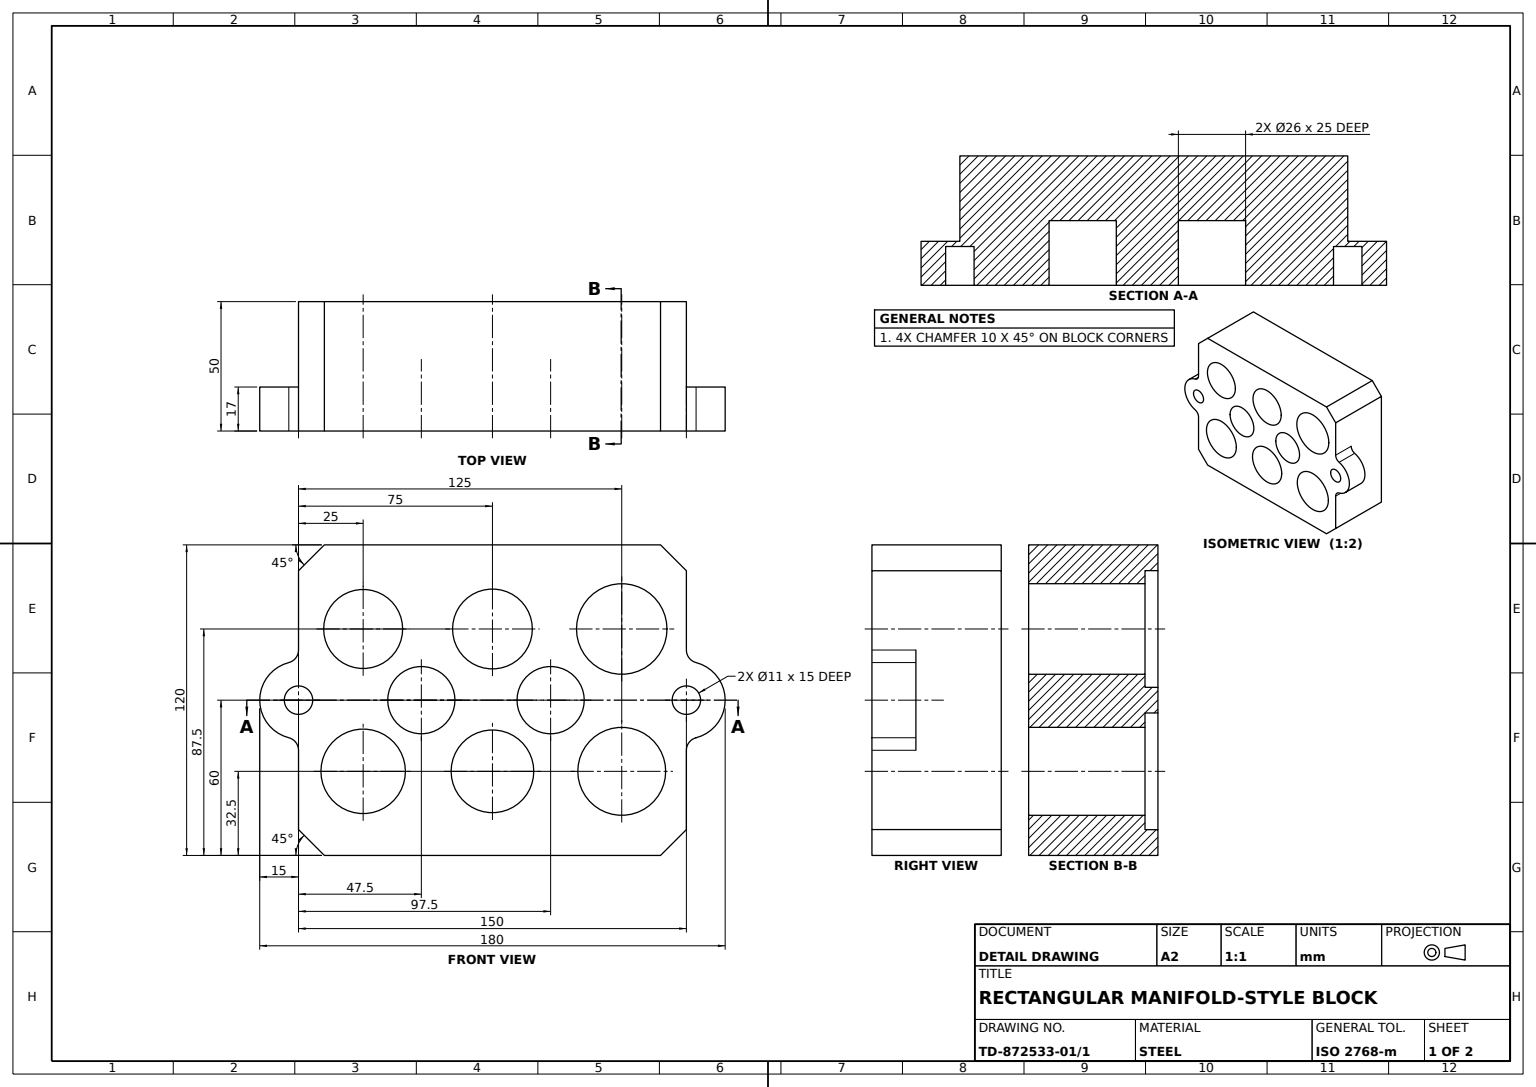
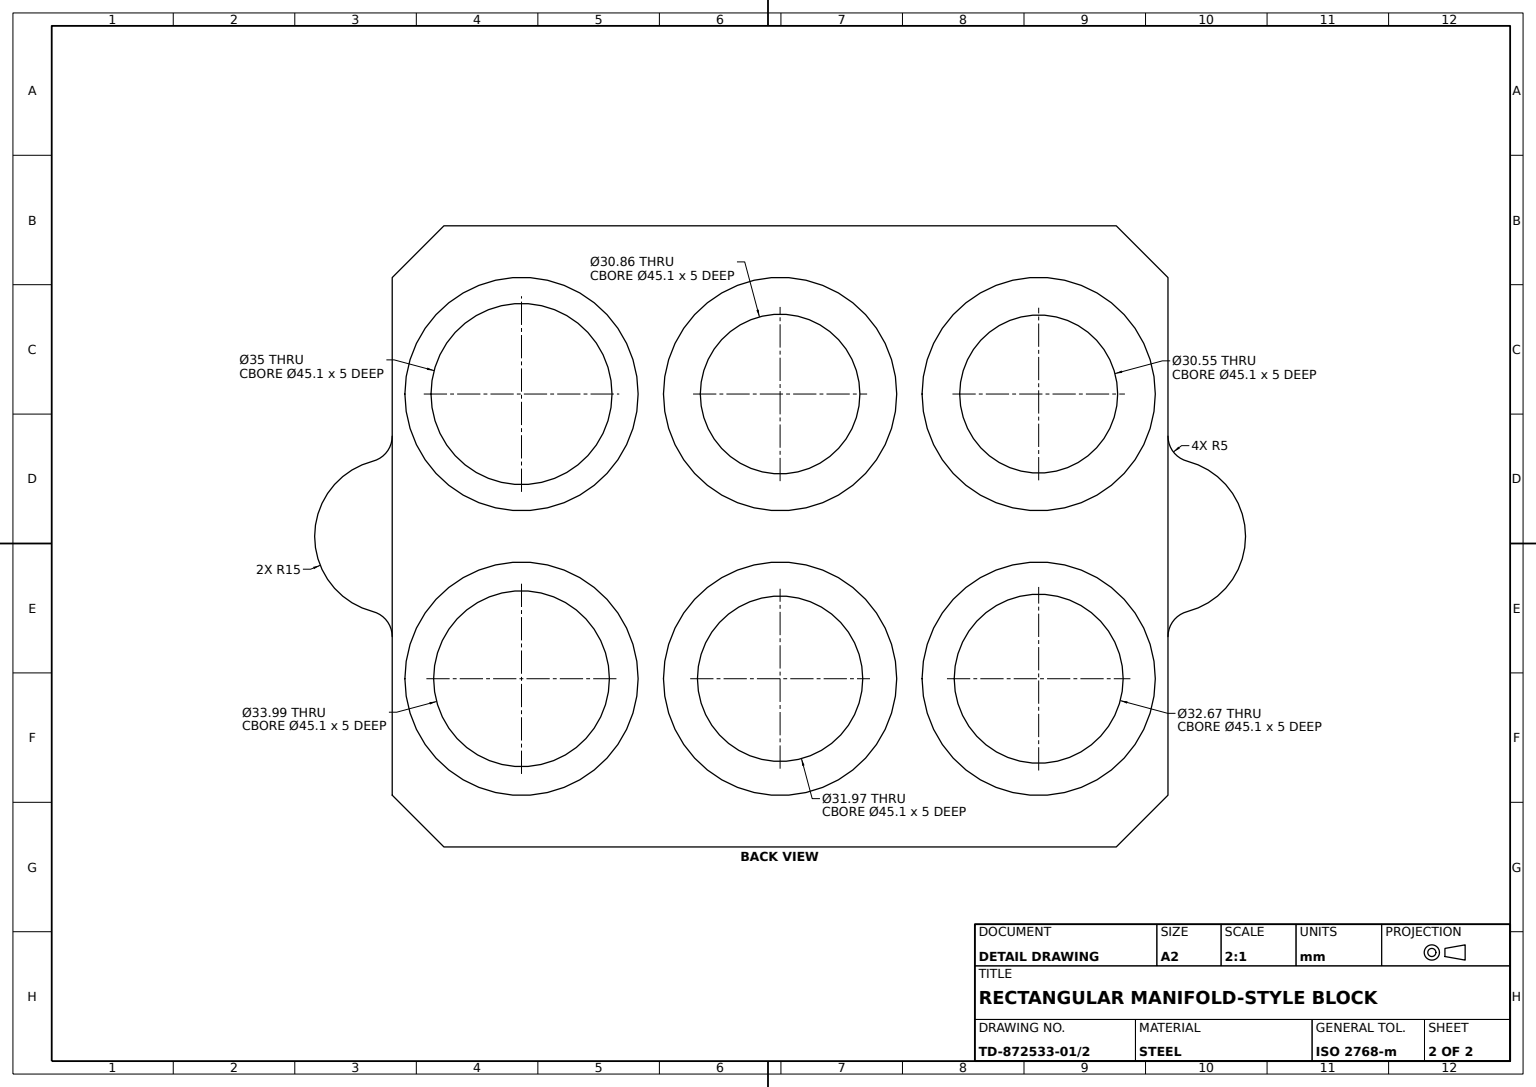
solid
v1 (153.75,74.523688,33)
v2 (150,79.364917,33)
e1 v1 v2 CIRCLE(AX(P(155,79.364917,33),D(0,0,-1),D(-1,0,0)),5)
v3 (165,60,33)
e2 v3 v1 CIRCLE(AX(P(150,60,33),D(0,0,1),D(-1,0,0)),15)
v4 (153.75,45.476312,33)
e3 v4 v3 CIRCLE(AX(P(150,60,33),D(0,0,1),D(-1,0,0)),15)
v5 (150,40.635083,33)
e4 v5 v4 CIRCLE(AX(P(155,40.635083,33),D(0,0,-1),D(1,0,0)),5)
e5 v2 v5 LINE
face PLANE(AX(P(150,60,33),D(0,0,-1),D(-1,0,0))) [-e1 -e2 -e3 -e4 -e5]
v6 (150,79.364917,50)
e6 v2 v6 LINE
v7 (150,40.635083,50)
e7 v5 v7 LINE
v8 (150,10,50)
e8 v8 v7 LINE
v9 (150,10,0)
e9 v8 v9 LINE
v10 (150,110,0)
e10 v9 v10 LINE
v11 (150,110,50)
e11 v10 v11 LINE
e12 v6 v11 LINE
face PLANE(AX(P(150,0,50),D(-1,0,0),D(0,0,1))) rev [-e6 e5 e7 -e8 e9 e10 e11 -e12]
v12 (142.5,87.5,50)
v13 (142.5,87.5,5)
e13 v12 v13 LINE
v14 (107.5,87.5,50)
e14 v14 v12 CIRCLE(AX(P(125,87.5,50),D(0,0,-1),D(-1,0,0)),17.5)
v15 (107.5,87.5,5)
e15 v14 v15 LINE
e16 v15 v13 CIRCLE(AX(P(125,87.5,5),D(0,0,-1),D(-1,0,0)),17.5)
face CYL(AX(P(125,87.5,50),D(0,0,-1),D(-1,0,0)),17.5) rev [-e13 -e14 e15 e16]
v16 (-5.5,60,35)
v17 (5.5,60,35)
e17 v16 v17 CIRCLE(AX(P(0,60,35),D(0,0,1),D(1,0,0)),5.5)
e18 v17 v16 CIRCLE(AX(P(0,60,35),D(0,0,1),D(1,0,0)),5.5)
face PLANE(AX(P(0,60,35),D(0,0,1),D(1,0,0))) [e17 e18]
v18 (2.45,87.5,5)
v19 (2.45,87.5,0)
e19 v18 v19 LINE
v20 (47.55,87.5,0)
e20 v19 v20 CIRCLE(AX(P(25,87.5,0),D(0,0,-1),D(-1,0,0)),22.55)
v21 (47.55,87.5,5)
e21 v21 v20 LINE
e22 v18 v21 CIRCLE(AX(P(25,87.5,5),D(0,0,-1),D(-1,0,0)),22.55)
face CYL(AX(P(25,87.5,5),D(0,0,-1),D(-1,0,0)),22.55) rev [e19 e20 -e21 -e22]
v22 (141.993107,32.5,50)
v23 (108.006893,32.5,50)
e23 v22 v23 CIRCLE(AX(P(125,32.5,50),D(0,0,-1),D(-1,0,0)),16.993107)
v24 (141.993107,32.5,5)
e24 v22 v24 LINE
v25 (108.006893,32.5,5)
e25 v24 v25 CIRCLE(AX(P(125,32.5,5),D(0,0,-1),D(-1,0,0)),16.993107)
e26 v23 v25 LINE
face CYL(AX(P(125,32.5,50),D(0,0,-1),D(-1,0,0)),16.993107) rev [-e23 e24 e25 -e26]
v26 (9.725741,87.5,50)
v27 (40.274259,87.5,50)
e27 v26 v27 CIRCLE(AX(P(25,87.5,50),D(0,0,-1),D(-1,0,0)),15.274259)
v28 (9.725741,87.5,5)
e28 v26 v28 LINE
v29 (40.274259,87.5,5)
e29 v28 v29 CIRCLE(AX(P(25,87.5,5),D(0,0,-1),D(-1,0,0)),15.274259)
e30 v27 v29 LINE
face CYL(AX(P(25,87.5,50),D(0,0,-1),D(-1,0,0)),15.274259) rev [-e27 e28 e29 -e30]
v30 (2.45,32.5,0)
v31 (47.55,32.5,0)
e31 v30 v31 CIRCLE(AX(P(25,32.5,0),D(0,0,-1),D(-1,0,0)),22.55)
v32 (47.55,32.5,5)
e32 v32 v31 LINE
v33 (2.45,32.5,5)
e33 v33 v32 CIRCLE(AX(P(25,32.5,5),D(0,0,-1),D(-1,0,0)),22.55)
e34 v33 v30 LINE
face CYL(AX(P(25,32.5,5),D(0,0,-1),D(-1,0,0)),22.55) rev [e31 -e32 -e33 e34]
v34 (110.5,60,25)
v35 (110.5,60,50)
e35 v34 v35 LINE
v36 (84.5,60,25)
e36 v36 v34 CIRCLE(AX(P(97.5,60,25),D(0,0,1),D(1,0,0)),13)
v37 (84.5,60,50)
e37 v36 v37 LINE
e38 v37 v35 CIRCLE(AX(P(97.5,60,50),D(0,0,1),D(1,0,0)),13)
face CYL(AX(P(97.5,60,25),D(0,0,1),D(1,0,0)),13) rev [-e35 -e36 e37 e38]
v38 (5.5,60,50)
e39 v17 v38 LINE
v39 (-5.5,60,50)
e40 v38 v39 CIRCLE(AX(P(0,60,50),D(0,0,1),D(1,0,0)),5.5)
e41 v16 v39 LINE
face CYL(AX(P(0,60,35),D(0,0,1),D(1,0,0)),5.5) rev [-e18 e39 e40 -e41]
v40 (102.45,87.5,5)
v41 (147.55,87.5,5)
e42 v40 v41 CIRCLE(AX(P(125,87.5,5),D(0,0,-1),D(-1,0,0)),22.55)
v42 (102.45,87.5,0)
e43 v40 v42 LINE
v43 (147.55,87.5,0)
e44 v42 v43 CIRCLE(AX(P(125,87.5,0),D(0,0,-1),D(-1,0,0)),22.55)
e45 v41 v43 LINE
face CYL(AX(P(125,87.5,5),D(0,0,-1),D(-1,0,0)),22.55) rev [-e42 e43 e44 -e45]
e46 v25 v24 CIRCLE(AX(P(125,32.5,5),D(0,0,-1),D(-1,0,0)),16.993107)
v44 (102.45,32.5,5)
v45 (147.55,32.5,5)
e47 v44 v45 CIRCLE(AX(P(125,32.5,5),D(0,0,-1),D(-1,0,0)),22.55)
e48 v45 v44 CIRCLE(AX(P(125,32.5,5),D(0,0,-1),D(-1,0,0)),22.55)
face PLANE(AX(P(125,32.5,5),D(0,0,-1),D(-1,0,0))) [-e46 -e25] [e47 e48]
v46 (52.45,87.5,5)
v47 (97.55,87.5,5)
e49 v46 v47 CIRCLE(AX(P(75,87.5,5),D(0,0,-1),D(-1,0,0)),22.55)
v48 (52.45,87.5,0)
e50 v46 v48 LINE
v49 (97.55,87.5,0)
e51 v48 v49 CIRCLE(AX(P(75,87.5,0),D(0,0,-1),D(-1,0,0)),22.55)
e52 v47 v49 LINE
face CYL(AX(P(75,87.5,5),D(0,0,-1),D(-1,0,0)),22.55) rev [-e49 e50 e51 -e52]
v50 (60.5,60,25)
v51 (34.5,60,25)
e53 v50 v51 CIRCLE(AX(P(47.5,60,25),D(0,0,1),D(1,0,0)),13)
e54 v51 v50 CIRCLE(AX(P(47.5,60,25),D(0,0,1),D(1,0,0)),13)
face PLANE(AX(P(47.5,60,25),D(0,0,1),D(1,0,0))) [e53 e54]
v52 (153.75,45.476312,50)
v53 (165,60,50)
e55 v52 v53 CIRCLE(AX(P(150,60,50),D(0,0,1),D(-1,0,0)),15)
e56 v4 v52 LINE
e57 v3 v53 LINE
face CYL(AX(P(150,60,33),D(0,0,1),D(1,0,0)),15) [-e55 -e56 e3 e57]
v54 (144.5,60,35)
v55 (155.5,60,35)
e58 v54 v55 CIRCLE(AX(P(150,60,35),D(0,0,1),D(1,0,0)),5.5)
v56 (144.5,60,50)
e59 v54 v56 LINE
v57 (155.5,60,50)
e60 v56 v57 CIRCLE(AX(P(150,60,50),D(0,0,1),D(1,0,0)),5.5)
e61 v55 v57 LINE
face CYL(AX(P(150,60,35),D(0,0,1),D(1,0,0)),5.5) rev [-e58 e59 e60 -e61]
v58 (90.429011,87.5,5)
v59 (59.570989,87.5,5)
e62 v58 v59 CIRCLE(AX(P(75,87.5,5),D(0,0,-1),D(-1,0,0)),15.429011)
e63 v59 v58 CIRCLE(AX(P(75,87.5,5),D(0,0,-1),D(-1,0,0)),15.429011)
e64 v47 v46 CIRCLE(AX(P(75,87.5,5),D(0,0,-1),D(-1,0,0)),22.55)
face PLANE(AX(P(75,87.5,5),D(0,0,-1),D(-1,0,0))) [-e62 -e63] [e64 e49]
v60 (0,110,50)
v61 (0,110,0)
e65 v60 v61 LINE
v62 (10,120,50)
e66 v62 v60 LINE
v63 (10,120,0)
e67 v63 v62 LINE
e68 v61 v63 LINE
face PLANE(AX(P(0,110,50),D(0.707106781,-0.707106781,0),D(0,0,-1))) rev [-e65 -e66 -e67 -e68]
v64 (140,120,0)
e69 v64 v63 LINE
v65 (140,120,50)
e70 v65 v62 LINE
e71 v65 v64 LINE
face PLANE(AX(P(0,120,50),D(0,-1,0),D(0,0,-1))) rev [e69 e67 -e70 e71]
v66 (8.666376,32.5,5)
v67 (41.333624,32.5,5)
e72 v66 v67 CIRCLE(AX(P(25,32.5,5),D(0,0,-1),D(-1,0,0)),16.333624)
v68 (41.333624,32.5,50)
e73 v68 v67 LINE
v69 (8.666376,32.5,50)
e74 v69 v68 CIRCLE(AX(P(25,32.5,50),D(0,0,-1),D(-1,0,0)),16.333624)
e75 v69 v66 LINE
face CYL(AX(P(25,32.5,50),D(0,0,-1),D(-1,0,0)),16.333624) rev [e72 -e73 -e74 e75]
v70 (90.982646,32.5,5)
v71 (59.017354,32.5,5)
e76 v70 v71 CIRCLE(AX(P(75,32.5,5),D(0,0,-1),D(-1,0,0)),15.982646)
v72 (59.017354,32.5,50)
e77 v72 v71 LINE
v73 (90.982646,32.5,50)
e78 v73 v72 CIRCLE(AX(P(75,32.5,50),D(0,0,-1),D(-1,0,0)),15.982646)
e79 v73 v70 LINE
face CYL(AX(P(75,32.5,50),D(0,0,-1),D(-1,0,0)),15.982646) rev [e76 -e77 -e78 e79]
v74 (60.5,60,50)
e80 v50 v74 LINE
v75 (34.5,60,50)
e81 v74 v75 CIRCLE(AX(P(47.5,60,50),D(0,0,1),D(1,0,0)),13)
e82 v51 v75 LINE
face CYL(AX(P(47.5,60,25),D(0,0,1),D(1,0,0)),13) rev [-e53 e80 e81 -e82]
e83 v55 v54 CIRCLE(AX(P(150,60,35),D(0,0,1),D(1,0,0)),5.5)
face PLANE(AX(P(150,60,35),D(0,0,1),D(1,0,0))) [e83 e58]
v76 (90.429011,87.5,50)
e84 v76 v58 LINE
v77 (59.570989,87.5,50)
e85 v77 v59 LINE
e86 v76 v77 CIRCLE(AX(P(75,87.5,50),D(0,0,-1),D(-1,0,0)),15.429011)
face CYL(AX(P(75,87.5,50),D(0,0,-1),D(-1,0,0)),15.429011) rev [e84 e62 -e85 -e86]
e87 v7 v52 CIRCLE(AX(P(155,40.635083,50),D(0,0,-1),D(1,0,0)),5)
face CYL(AX(P(155,40.635083,33),D(0,0,1),D(1,0,0)),5) rev [e56 -e87 -e7 e4]
v78 (0,10,0)
v79 (0,10,50)
e88 v78 v79 LINE
v80 (10,0,0)
e89 v80 v78 LINE
v81 (10,0,50)
e90 v81 v80 LINE
e91 v79 v81 LINE
face PLANE(AX(P(10,0,50),D(0.707106781,0.707106781,0),D(0,0,-1))) rev [-e88 -e89 -e90 -e91]
e92 v77 v76 CIRCLE(AX(P(75,87.5,50),D(0,0,-1),D(-1,0,0)),15.429011)
face CYL(AX(P(75,87.5,50),D(0,0,-1),D(-1,0,0)),15.429011) rev [-e84 -e92 e85 e63]
e93 v27 v26 CIRCLE(AX(P(25,87.5,50),D(0,0,-1),D(-1,0,0)),15.274259)
e94 v29 v28 CIRCLE(AX(P(25,87.5,5),D(0,0,-1),D(-1,0,0)),15.274259)
face CYL(AX(P(25,87.5,50),D(0,0,-1),D(-1,0,0)),15.274259) rev [-e93 e30 e94 -e28]
e95 v12 v14 CIRCLE(AX(P(125,87.5,50),D(0,0,-1),D(-1,0,0)),17.5)
e96 v39 v38 CIRCLE(AX(P(0,60,50),D(0,0,1),D(1,0,0)),5.5)
e97 v75 v74 CIRCLE(AX(P(47.5,60,50),D(0,0,1),D(1,0,0)),13)
e98 v35 v37 CIRCLE(AX(P(97.5,60,50),D(0,0,1),D(1,0,0)),13)
v82 (-3.75,45.476312,50)
v83 (0,40.635083,50)
e99 v82 v83 CIRCLE(AX(P(-5,40.635083,50),D(0,0,-1),D(-1,0,0)),5)
e100 v83 v79 LINE
v84 (140,0,50)
e101 v81 v84 LINE
e102 v84 v8 LINE
v85 (153.75,74.523688,50)
e103 v53 v85 CIRCLE(AX(P(150,60,50),D(0,0,1),D(-1,0,0)),15)
e104 v85 v6 CIRCLE(AX(P(155,79.364917,50),D(0,0,-1),D(-1,0,0)),5)
e105 v11 v65 LINE
v86 (0,79.364917,50)
e106 v60 v86 LINE
v87 (-3.75,74.523688,50)
e107 v86 v87 CIRCLE(AX(P(-5,79.364917,50),D(0,0,-1),D(1,0,0)),5)
e108 v87 v82 CIRCLE(AX(P(0,60,50),D(0,0,1),D(1,0,0)),15)
e109 v72 v73 CIRCLE(AX(P(75,32.5,50),D(0,0,-1),D(-1,0,0)),15.982646)
e110 v68 v69 CIRCLE(AX(P(25,32.5,50),D(0,0,-1),D(-1,0,0)),16.333624)
e111 v23 v22 CIRCLE(AX(P(125,32.5,50),D(0,0,-1),D(-1,0,0)),16.993107)
e112 v57 v56 CIRCLE(AX(P(150,60,50),D(0,0,1),D(1,0,0)),5.5)
face PLANE(AX(P(0,0,50),D(0,0,-1),D(-1,0,0))) rev [e95 e14] [-e96 -e40] [-e97 -e81] [-e38 -e98] [e99 e100 e91 e101 e102 e8 e87 e55 e103 e104 e12 e105 e70 e66 e106 e107 e108] [e109 e78] [e74 e110] [e23 e111] [-e60 -e112] [e93 e27] [e86 e92]
e113 v1 v85 LINE
face CYL(AX(P(155,79.364917,33),D(0,0,1),D(1,0,0)),5) rev [e1 e6 -e104 -e113]
v88 (140,0,0)
e114 v88 v84 LINE
e115 v9 v88 LINE
face PLANE(AX(P(150,10,50),D(-0.707106781,0.707106781,0),D(0,0,-1))) rev [-e102 -e114 -e115 -e9]
v89 (0,79.364917,33)
v90 (-3.75,74.523688,33)
e116 v89 v90 CIRCLE(AX(P(-5,79.364917,33),D(0,0,-1),D(1,0,0)),5)
v91 (0,40.635083,33)
e117 v91 v89 LINE
v92 (-3.75,45.476312,33)
e118 v92 v91 CIRCLE(AX(P(-5,40.635083,33),D(0,0,-1),D(-1,0,0)),5)
e119 v90 v92 CIRCLE(AX(P(0,60,33),D(0,0,1),D(1,0,0)),15)
face PLANE(AX(P(-5,79.364917,33),D(0,0,1),D(1,0,0))) rev [-e116 -e117 -e118 -e119]
e120 v64 v10 LINE
e121 v80 v88 LINE
e122 v61 v78 LINE
v93 (147.55,32.5,0)
v94 (102.45,32.5,0)
e123 v93 v94 CIRCLE(AX(P(125,32.5,0),D(0,0,-1),D(-1,0,0)),22.55)
e124 v94 v93 CIRCLE(AX(P(125,32.5,0),D(0,0,-1),D(-1,0,0)),22.55)
e125 v43 v42 CIRCLE(AX(P(125,87.5,0),D(0,0,-1),D(-1,0,0)),22.55)
v95 (97.55,32.5,0)
v96 (52.45,32.5,0)
e126 v95 v96 CIRCLE(AX(P(75,32.5,0),D(0,0,-1),D(-1,0,0)),22.55)
e127 v96 v95 CIRCLE(AX(P(75,32.5,0),D(0,0,-1),D(-1,0,0)),22.55)
e128 v31 v30 CIRCLE(AX(P(25,32.5,0),D(0,0,-1),D(-1,0,0)),22.55)
e129 v20 v19 CIRCLE(AX(P(25,87.5,0),D(0,0,-1),D(-1,0,0)),22.55)
e130 v49 v48 CIRCLE(AX(P(75,87.5,0),D(0,0,-1),D(-1,0,0)),22.55)
face PLANE(AX(P(0,0,0),D(0,0,-1),D(-1,0,0))) [e68 -e69 e120 -e10 e115 -e121 e89 -e122] [-e123 -e124] [-e44 -e125] [-e126 -e127] [-e31 -e128] [-e129 -e20] [-e130 -e51]
e131 v34 v36 CIRCLE(AX(P(97.5,60,25),D(0,0,1),D(1,0,0)),13)
face CYL(AX(P(97.5,60,25),D(0,0,1),D(1,0,0)),13) rev [-e131 e35 e98 -e37]
v97 (97.55,32.5,5)
e132 v97 v95 LINE
v98 (52.45,32.5,5)
e133 v98 v96 LINE
e134 v97 v98 CIRCLE(AX(P(75,32.5,5),D(0,0,-1),D(-1,0,0)),22.55)
face CYL(AX(P(75,32.5,5),D(0,0,-1),D(-1,0,0)),22.55) rev [e132 e126 -e133 -e134]
e135 v90 v87 LINE
e136 v89 v86 LINE
face CYL(AX(P(-5,79.364917,33),D(0,0,1),D(1,0,0)),5) rev [e116 e135 -e107 -e136]
e137 v71 v70 CIRCLE(AX(P(75,32.5,5),D(0,0,-1),D(-1,0,0)),15.982646)
face CYL(AX(P(75,32.5,50),D(0,0,-1),D(-1,0,0)),15.982646) rev [-e109 e77 e137 -e79]
e138 v32 v33 CIRCLE(AX(P(25,32.5,5),D(0,0,-1),D(-1,0,0)),22.55)
e139 v67 v66 CIRCLE(AX(P(25,32.5,5),D(0,0,-1),D(-1,0,0)),16.333624)
face PLANE(AX(P(25,32.5,5),D(0,0,-1),D(-1,0,0))) [e138 e33] [-e72 -e139]
e140 v92 v82 LINE
face CYL(AX(P(0,60,33),D(0,0,1),D(1,0,0)),15) [-e108 -e135 e119 e140]
e141 v13 v15 CIRCLE(AX(P(125,87.5,5),D(0,0,-1),D(-1,0,0)),17.5)
e142 v41 v40 CIRCLE(AX(P(125,87.5,5),D(0,0,-1),D(-1,0,0)),22.55)
face PLANE(AX(P(125,87.5,5),D(0,0,-1),D(-1,0,0))) [-e16 -e141] [e42 e142]
e143 v98 v97 CIRCLE(AX(P(75,32.5,5),D(0,0,-1),D(-1,0,0)),22.55)
face CYL(AX(P(75,32.5,5),D(0,0,-1),D(-1,0,0)),22.55) rev [-e143 e133 e127 -e132]
face CYL(AX(P(25,32.5,50),D(0,0,-1),D(-1,0,0)),16.333624) rev [e73 e139 -e75 -e110]
face CYL(AX(P(150,60,35),D(0,0,1),D(1,0,0)),5.5) rev [-e59 -e83 e61 e112]
face CYL(AX(P(125,32.5,50),D(0,0,-1),D(-1,0,0)),16.993107) rev [-e111 e26 e46 -e24]
e144 v21 v18 CIRCLE(AX(P(25,87.5,5),D(0,0,-1),D(-1,0,0)),22.55)
face PLANE(AX(P(25,87.5,5),D(0,0,-1),D(-1,0,0))) [e22 e144] [-e94 -e29]
face CYL(AX(P(47.5,60,25),D(0,0,1),D(1,0,0)),13) rev [-e80 -e54 e82 e97]
e145 v91 v83 LINE
face CYL(AX(P(-5,40.635083,33),D(0,0,1),D(1,0,0)),5) rev [e118 e145 -e99 -e140]
face CYL(AX(P(75,87.5,5),D(0,0,-1),D(-1,0,0)),22.55) rev [e52 e130 -e50 -e64]
face CYL(AX(P(25,32.5,5),D(0,0,-1),D(-1,0,0)),22.55) rev [e128 -e34 -e138 e32]
face CYL(AX(P(150,60,33),D(0,0,1),D(1,0,0)),15) [e113 -e103 -e57 e2]
face PLANE(AX(P(97.5,60,25),D(0,0,1),D(1,0,0))) [e36 e131]
face PLANE(AX(P(140,120,50),D(-0.707106781,-0.707106781,0),D(0,0,-1))) rev [-e11 -e120 -e71 -e105]
face PLANE(AX(P(75,32.5,5),D(0,0,-1),D(-1,0,0))) [e134 e143] [-e137 -e76]
face CYL(AX(P(125,87.5,50),D(0,0,-1),D(-1,0,0)),17.5) rev [e13 e141 -e15 -e95]
e146 v45 v93 LINE
e147 v44 v94 LINE
face CYL(AX(P(125,32.5,5),D(0,0,-1),D(-1,0,0)),22.55) rev [-e48 e146 e123 -e147]
face PLANE(AX(P(0,0,50),D(0,1,0),D(0,0,1))) rev [e121 e114 -e101 e90]
face PLANE(AX(P(0,0,50),D(1,0,0),D(0,0,-1))) rev [e117 e136 -e106 e65 e122 e88 -e100 -e145]
face CYL(AX(P(0,60,35),D(0,0,1),D(1,0,0)),5.5) rev [-e17 e41 e96 -e39]
face CYL(AX(P(125,87.5,5),D(0,0,-1),D(-1,0,0)),22.55) rev [e125 -e43 -e142 e45]
face CYL(AX(P(25,87.5,5),D(0,0,-1),D(-1,0,0)),22.55) rev [e129 -e19 -e144 e21]
face CYL(AX(P(125,32.5,5),D(0,0,-1),D(-1,0,0)),22.55) rev [e124 -e146 -e47 e147]
